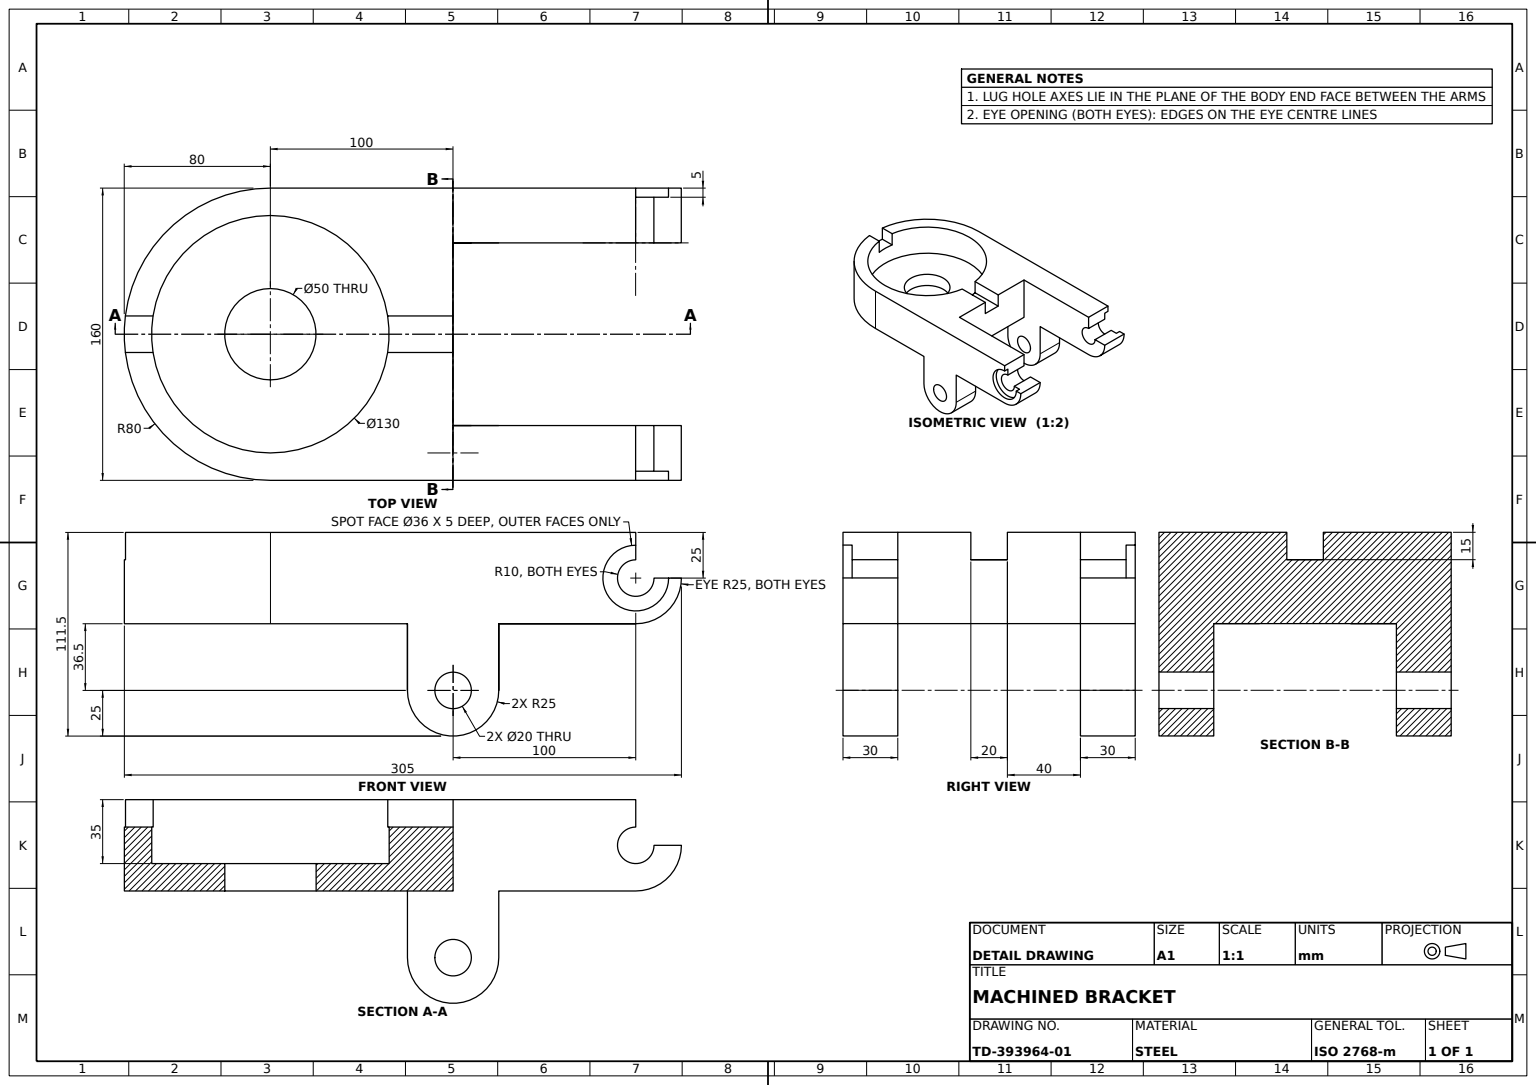
ISO-10303-21;
HEADER;
FILE_DESCRIPTION((''),'2;1');
FILE_NAME('','',(''),(''),'','','');
FILE_SCHEMA(('AUTOMOTIVE_DESIGN'));
ENDSEC;
DATA;
#1=APPLICATION_CONTEXT('');
#2=PRODUCT_CONTEXT('',#1,'mechanical');
#3=PRODUCT('','','',(#2));
#4=PRODUCT_DEFINITION_FORMATION('','',#3);
#5=PRODUCT_DEFINITION_CONTEXT('',#1,'design');
#6=PRODUCT_DEFINITION('','',#4,#5);
#7=PRODUCT_DEFINITION_SHAPE('','',#6);
#8=(LENGTH_UNIT()NAMED_UNIT(*)SI_UNIT(.MILLI.,.METRE.));
#9=(NAMED_UNIT(*)PLANE_ANGLE_UNIT()SI_UNIT($,.RADIAN.));
#10=(NAMED_UNIT(*)SI_UNIT($,.STERADIAN.)SOLID_ANGLE_UNIT());
#11=UNCERTAINTY_MEASURE_WITH_UNIT(LENGTH_MEASURE(1.E-05),#8,'distance_accuracy_value','');
#12=(GEOMETRIC_REPRESENTATION_CONTEXT(3)GLOBAL_UNCERTAINTY_ASSIGNED_CONTEXT((#11))GLOBAL_UNIT_ASSIGNED_CONTEXT((#8,#9,#10))REPRESENTATION_CONTEXT('',''));
#13=CARTESIAN_POINT('',(75.,-35.,50.));
#14=VERTEX_POINT('',#13);
#15=CARTESIAN_POINT('',(100.,-35.,50.));
#16=VERTEX_POINT('',#15);
#17=CARTESIAN_POINT('',(0.,-35.,50.));
#18=DIRECTION('',(1.,0.,0.));
#19=VECTOR('',#18,1000.);
#20=LINE('',#17,#19);
#21=EDGE_CURVE('',#14,#16,#20,.T.);
#22=ORIENTED_EDGE('',*,*,#21,.F.);
#23=CARTESIAN_POINT('',(75.,-35.,80.));
#24=VERTEX_POINT('',#23);
#25=DIRECTION('',(0.,0.,1.));
#26=VECTOR('',#25,1000.);
#27=LINE('',#13,#26);
#28=EDGE_CURVE('',#14,#24,#27,.T.);
#29=ORIENTED_EDGE('',*,*,#28,.T.);
#30=CARTESIAN_POINT('',(0.,-35.,80.));
#31=VERTEX_POINT('',#30);
#32=DIRECTION('',(-1.,0.,0.));
#33=VECTOR('',#32,1000.);
#34=LINE('',#30,#33);
#35=EDGE_CURVE('',#24,#31,#34,.T.);
#36=ORIENTED_EDGE('',*,*,#35,.T.);
#37=CARTESIAN_POINT('',(0.,-35.,-80.));
#38=VERTEX_POINT('',#37);
#39=CARTESIAN_POINT('',(0.,-35.,0.));
#40=DIRECTION('',(0.,-1.,0.));
#41=DIRECTION('',(0.,0.,-1.));
#42=AXIS2_PLACEMENT_3D('',#39,#40,#41);
#43=CIRCLE('',#42,80.);
#44=EDGE_CURVE('',#31,#38,#43,.T.);
#45=ORIENTED_EDGE('',*,*,#44,.T.);
#46=CARTESIAN_POINT('',(75.,-35.,-80.));
#47=VERTEX_POINT('',#46);
#48=LINE('',#37,#33);
#49=EDGE_CURVE('',#47,#38,#48,.T.);
#50=ORIENTED_EDGE('',*,*,#49,.F.);
#51=CARTESIAN_POINT('',(75.,-35.,-50.));
#52=VERTEX_POINT('',#51);
#53=VECTOR('',#41,1000.);
#54=LINE('',#51,#53);
#55=EDGE_CURVE('',#52,#47,#54,.T.);
#56=ORIENTED_EDGE('',*,*,#55,.F.);
#57=CARTESIAN_POINT('',(100.,-35.,-50.));
#58=VERTEX_POINT('',#57);
#59=CARTESIAN_POINT('',(0.,-35.,-50.));
#60=LINE('',#59,#19);
#61=EDGE_CURVE('',#52,#58,#60,.T.);
#62=ORIENTED_EDGE('',*,*,#61,.T.);
#63=CARTESIAN_POINT('',(100.,-35.,0.));
#64=LINE('',#63,#26);
#65=EDGE_CURVE('',#58,#16,#64,.T.);
#66=ORIENTED_EDGE('',*,*,#65,.T.);
#67=EDGE_LOOP('',(#22,#29,#36,#45,#50,#56,#62,#66));
#68=FACE_OUTER_BOUND('',#67,.T.);
#69=CARTESIAN_POINT('',(0.,-35.,25.));
#70=VERTEX_POINT('',#69);
#71=CARTESIAN_POINT('',(0.,-35.,-25.));
#72=VERTEX_POINT('',#71);
#73=CIRCLE('',#42,25.);
#74=EDGE_CURVE('',#70,#72,#73,.T.);
#75=ORIENTED_EDGE('',*,*,#74,.F.);
#76=EDGE_CURVE('',#72,#70,#73,.T.);
#77=ORIENTED_EDGE('',*,*,#76,.F.);
#78=EDGE_LOOP('',(#75,#77));
#79=FACE_BOUND('',#78,.T.);
#80=PLANE('',#42);
#81=ADVANCED_FACE('',(#68,#79),#80,.T.);
#82=CARTESIAN_POINT('',(0.,-20.,-65.));
#83=VERTEX_POINT('',#82);
#84=CARTESIAN_POINT('',(0.,-20.,65.));
#85=VERTEX_POINT('',#84);
#86=CARTESIAN_POINT('',(0.,-20.,0.));
#87=AXIS2_PLACEMENT_3D('',#86,#40,#41);
#88=CIRCLE('',#87,65.);
#89=EDGE_CURVE('',#83,#85,#88,.T.);
#90=ORIENTED_EDGE('',*,*,#89,.T.);
#91=CARTESIAN_POINT('',(0.,15.,65.));
#92=VERTEX_POINT('',#91);
#93=VECTOR('',#40,1000.);
#94=LINE('',#91,#93);
#95=EDGE_CURVE('',#92,#85,#94,.T.);
#96=ORIENTED_EDGE('',*,*,#95,.F.);
#97=CARTESIAN_POINT('',(64.226163,15.,10.));
#98=VERTEX_POINT('',#97);
#99=CARTESIAN_POINT('',(0.,15.,0.));
#100=DIRECTION('',(0.,1.,0.));
#101=AXIS2_PLACEMENT_3D('',#99,#100,#25);
#102=CIRCLE('',#101,65.);
#103=EDGE_CURVE('',#92,#98,#102,.T.);
#104=ORIENTED_EDGE('',*,*,#103,.T.);
#105=CARTESIAN_POINT('',(64.226163,0.,10.));
#106=VERTEX_POINT('',#105);
#107=LINE('',#97,#93);
#108=EDGE_CURVE('',#98,#106,#107,.T.);
#109=ORIENTED_EDGE('',*,*,#108,.T.);
#110=CARTESIAN_POINT('',(64.226163,0.,-10.));
#111=VERTEX_POINT('',#110);
#112=CARTESIAN_POINT('',(0.,0.,0.));
#113=AXIS2_PLACEMENT_3D('',#112,#100,#41);
#114=CIRCLE('',#113,65.);
#115=EDGE_CURVE('',#106,#111,#114,.T.);
#116=ORIENTED_EDGE('',*,*,#115,.T.);
#117=CARTESIAN_POINT('',(64.226163,15.,-10.));
#118=VERTEX_POINT('',#117);
#119=LINE('',#117,#93);
#120=EDGE_CURVE('',#118,#111,#119,.T.);
#121=ORIENTED_EDGE('',*,*,#120,.F.);
#122=CARTESIAN_POINT('',(0.,15.,-65.));
#123=VERTEX_POINT('',#122);
#124=EDGE_CURVE('',#118,#123,#102,.T.);
#125=ORIENTED_EDGE('',*,*,#124,.T.);
#126=LINE('',#122,#93);
#127=EDGE_CURVE('',#123,#83,#126,.T.);
#128=ORIENTED_EDGE('',*,*,#127,.T.);
#129=EDGE_LOOP('',(#90,#96,#104,#109,#116,#121,#125,#128));
#130=FACE_OUTER_BOUND('',#129,.T.);
#131=AXIS2_PLACEMENT_3D('',#99,#40,#41);
#132=CYLINDRICAL_SURFACE('',#131,65.);
#133=ADVANCED_FACE('',(#130),#132,.F.);
#134=CARTESIAN_POINT('',(90.,-71.5,80.));
#135=VERTEX_POINT('',#134);
#136=CARTESIAN_POINT('',(110.,-71.5,80.));
#137=VERTEX_POINT('',#136);
#138=CARTESIAN_POINT('',(100.,-71.5,80.));
#139=AXIS2_PLACEMENT_3D('',#138,#25,#18);
#140=CIRCLE('',#139,10.);
#141=EDGE_CURVE('',#135,#137,#140,.T.);
#142=ORIENTED_EDGE('',*,*,#141,.F.);
#143=EDGE_CURVE('',#137,#135,#140,.T.);
#144=ORIENTED_EDGE('',*,*,#143,.F.);
#145=EDGE_LOOP('',(#142,#144));
#146=FACE_BOUND('',#145,.T.);
#147=CARTESIAN_POINT('',(0.,15.,80.));
#148=VERTEX_POINT('',#147);
#149=CARTESIAN_POINT('',(200.,15.,80.));
#150=VERTEX_POINT('',#149);
#151=LINE('',#147,#19);
#152=EDGE_CURVE('',#148,#150,#151,.T.);
#153=ORIENTED_EDGE('',*,*,#152,.F.);
#154=VECTOR('',#100,1000.);
#155=LINE('',#30,#154);
#156=EDGE_CURVE('',#31,#148,#155,.T.);
#157=ORIENTED_EDGE('',*,*,#156,.F.);
#158=ORIENTED_EDGE('',*,*,#35,.F.);
#159=CARTESIAN_POINT('',(75.,-71.5,80.));
#160=VERTEX_POINT('',#159);
#161=CARTESIAN_POINT('',(75.,0.,80.));
#162=LINE('',#161,#154);
#163=EDGE_CURVE('',#160,#24,#162,.T.);
#164=ORIENTED_EDGE('',*,*,#163,.F.);
#165=CARTESIAN_POINT('',(125.,-71.5,80.));
#166=VERTEX_POINT('',#165);
#167=CIRCLE('',#139,25.);
#168=EDGE_CURVE('',#160,#166,#167,.T.);
#169=ORIENTED_EDGE('',*,*,#168,.T.);
#170=CARTESIAN_POINT('',(125.,-35.,80.));
#171=VERTEX_POINT('',#170);
#172=CARTESIAN_POINT('',(125.,0.,80.));
#173=LINE('',#172,#93);
#174=EDGE_CURVE('',#171,#166,#173,.T.);
#175=ORIENTED_EDGE('',*,*,#174,.F.);
#176=CARTESIAN_POINT('',(200.,-35.,80.));
#177=VERTEX_POINT('',#176);
#178=EDGE_CURVE('',#177,#171,#34,.T.);
#179=ORIENTED_EDGE('',*,*,#178,.F.);
#180=CARTESIAN_POINT('',(225.,-10.,80.));
#181=VERTEX_POINT('',#180);
#182=CARTESIAN_POINT('',(200.,-10.,80.));
#183=AXIS2_PLACEMENT_3D('',#182,#25,#18);
#184=CIRCLE('',#183,25.);
#185=EDGE_CURVE('',#177,#181,#184,.T.);
#186=ORIENTED_EDGE('',*,*,#185,.T.);
#187=CARTESIAN_POINT('',(218.,-10.,80.));
#188=VERTEX_POINT('',#187);
#189=LINE('',#182,#19);
#190=EDGE_CURVE('',#188,#181,#189,.T.);
#191=ORIENTED_EDGE('',*,*,#190,.F.);
#192=CARTESIAN_POINT('',(200.,8.,80.));
#193=VERTEX_POINT('',#192);
#194=CIRCLE('',#183,18.);
#195=EDGE_CURVE('',#193,#188,#194,.T.);
#196=ORIENTED_EDGE('',*,*,#195,.F.);
#197=LINE('',#149,#93);
#198=EDGE_CURVE('',#150,#193,#197,.T.);
#199=ORIENTED_EDGE('',*,*,#198,.F.);
#200=EDGE_LOOP('',(#153,#157,#158,#164,#169,#175,#179,#186,#191,#196,#199));
#201=FACE_OUTER_BOUND('',#200,.T.);
#202=AXIS2_PLACEMENT_3D('',#30,#41,#32);
#203=PLANE('',#202);
#204=ADVANCED_FACE('',(#146,#201),#203,.F.);
#205=ORIENTED_EDGE('',*,*,#127,.F.);
#206=CARTESIAN_POINT('',(-64.226163,15.,-10.));
#207=VERTEX_POINT('',#206);
#208=EDGE_CURVE('',#123,#207,#102,.T.);
#209=ORIENTED_EDGE('',*,*,#208,.T.);
#210=CARTESIAN_POINT('',(-64.226163,0.,-10.));
#211=VERTEX_POINT('',#210);
#212=LINE('',#206,#93);
#213=EDGE_CURVE('',#207,#211,#212,.T.);
#214=ORIENTED_EDGE('',*,*,#213,.T.);
#215=CARTESIAN_POINT('',(-64.226163,0.,10.));
#216=VERTEX_POINT('',#215);
#217=EDGE_CURVE('',#211,#216,#114,.T.);
#218=ORIENTED_EDGE('',*,*,#217,.T.);
#219=CARTESIAN_POINT('',(-64.226163,15.,10.));
#220=VERTEX_POINT('',#219);
#221=LINE('',#219,#93);
#222=EDGE_CURVE('',#220,#216,#221,.T.);
#223=ORIENTED_EDGE('',*,*,#222,.F.);
#224=EDGE_CURVE('',#220,#92,#102,.T.);
#225=ORIENTED_EDGE('',*,*,#224,.T.);
#226=ORIENTED_EDGE('',*,*,#95,.T.);
#227=EDGE_CURVE('',#85,#83,#88,.T.);
#228=ORIENTED_EDGE('',*,*,#227,.T.);
#229=EDGE_LOOP('',(#205,#209,#214,#218,#223,#225,#226,#228));
#230=FACE_OUTER_BOUND('',#229,.T.);
#231=ADVANCED_FACE('',(#230),#132,.F.);
#232=CARTESIAN_POINT('',(0.,-20.,25.));
#233=VERTEX_POINT('',#232);
#234=LINE('',#232,#93);
#235=EDGE_CURVE('',#233,#70,#234,.T.);
#236=ORIENTED_EDGE('',*,*,#235,.F.);
#237=CARTESIAN_POINT('',(0.,-20.,-25.));
#238=VERTEX_POINT('',#237);
#239=CIRCLE('',#87,25.);
#240=EDGE_CURVE('',#238,#233,#239,.T.);
#241=ORIENTED_EDGE('',*,*,#240,.F.);
#242=LINE('',#237,#93);
#243=EDGE_CURVE('',#238,#72,#242,.T.);
#244=ORIENTED_EDGE('',*,*,#243,.T.);
#245=ORIENTED_EDGE('',*,*,#76,.T.);
#246=EDGE_LOOP('',(#236,#241,#244,#245));
#247=FACE_OUTER_BOUND('',#246,.T.);
#248=CYLINDRICAL_SURFACE('',#87,25.);
#249=ADVANCED_FACE('',(#247),#248,.F.);
#250=CARTESIAN_POINT('',(125.,-71.5,-80.));
#251=VERTEX_POINT('',#250);
#252=CARTESIAN_POINT('',(75.,-71.5,-80.));
#253=VERTEX_POINT('',#252);
#254=CARTESIAN_POINT('',(100.,-71.5,-80.));
#255=AXIS2_PLACEMENT_3D('',#254,#41,#32);
#256=CIRCLE('',#255,25.);
#257=EDGE_CURVE('',#251,#253,#256,.T.);
#258=ORIENTED_EDGE('',*,*,#257,.F.);
#259=CARTESIAN_POINT('',(125.,-71.5,-50.));
#260=VERTEX_POINT('',#259);
#261=LINE('',#259,#53);
#262=EDGE_CURVE('',#260,#251,#261,.T.);
#263=ORIENTED_EDGE('',*,*,#262,.F.);
#264=CARTESIAN_POINT('',(75.,-71.5,-50.));
#265=VERTEX_POINT('',#264);
#266=CARTESIAN_POINT('',(100.,-71.5,-50.));
#267=AXIS2_PLACEMENT_3D('',#266,#41,#32);
#268=CIRCLE('',#267,25.);
#269=EDGE_CURVE('',#260,#265,#268,.T.);
#270=ORIENTED_EDGE('',*,*,#269,.T.);
#271=LINE('',#264,#53);
#272=EDGE_CURVE('',#265,#253,#271,.T.);
#273=ORIENTED_EDGE('',*,*,#272,.T.);
#274=EDGE_LOOP('',(#258,#263,#270,#273));
#275=FACE_OUTER_BOUND('',#274,.T.);
#276=CYLINDRICAL_SURFACE('',#267,25.);
#277=ADVANCED_FACE('',(#275),#276,.T.);
#278=CARTESIAN_POINT('',(90.,-71.5,50.));
#279=VERTEX_POINT('',#278);
#280=LINE('',#278,#26);
#281=EDGE_CURVE('',#279,#135,#280,.T.);
#282=ORIENTED_EDGE('',*,*,#281,.F.);
#283=CARTESIAN_POINT('',(110.,-71.5,50.));
#284=VERTEX_POINT('',#283);
#285=CARTESIAN_POINT('',(100.,-71.5,50.));
#286=AXIS2_PLACEMENT_3D('',#285,#25,#18);
#287=CIRCLE('',#286,10.);
#288=EDGE_CURVE('',#284,#279,#287,.T.);
#289=ORIENTED_EDGE('',*,*,#288,.F.);
#290=LINE('',#283,#26);
#291=EDGE_CURVE('',#284,#137,#290,.T.);
#292=ORIENTED_EDGE('',*,*,#291,.T.);
#293=ORIENTED_EDGE('',*,*,#143,.T.);
#294=EDGE_LOOP('',(#282,#289,#292,#293));
#295=FACE_OUTER_BOUND('',#294,.T.);
#296=CYLINDRICAL_SURFACE('',#286,10.);
#297=ADVANCED_FACE('',(#295),#296,.F.);
#298=CARTESIAN_POINT('',(125.,-35.,-50.));
#299=VERTEX_POINT('',#298);
#300=CARTESIAN_POINT('',(125.,-35.,-80.));
#301=VERTEX_POINT('',#300);
#302=LINE('',#298,#53);
#303=EDGE_CURVE('',#299,#301,#302,.T.);
#304=ORIENTED_EDGE('',*,*,#303,.T.);
#305=CARTESIAN_POINT('',(200.,-35.,-80.));
#306=VERTEX_POINT('',#305);
#307=EDGE_CURVE('',#306,#301,#48,.T.);
#308=ORIENTED_EDGE('',*,*,#307,.F.);
#309=CARTESIAN_POINT('',(200.,-35.,-50.));
#310=VERTEX_POINT('',#309);
#311=CARTESIAN_POINT('',(200.,-35.,0.));
#312=LINE('',#311,#53);
#313=EDGE_CURVE('',#310,#306,#312,.T.);
#314=ORIENTED_EDGE('',*,*,#313,.F.);
#315=EDGE_CURVE('',#299,#310,#60,.T.);
#316=ORIENTED_EDGE('',*,*,#315,.F.);
#317=EDGE_LOOP('',(#304,#308,#314,#316));
#318=FACE_OUTER_BOUND('',#317,.T.);
#319=ADVANCED_FACE('',(#318),#80,.T.);
#320=CARTESIAN_POINT('',(100.,15.,-10.));
#321=VERTEX_POINT('',#320);
#322=CARTESIAN_POINT('',(100.,0.,-10.));
#323=VERTEX_POINT('',#322);
#324=LINE('',#320,#93);
#325=EDGE_CURVE('',#321,#323,#324,.T.);
#326=ORIENTED_EDGE('',*,*,#325,.F.);
#327=CARTESIAN_POINT('',(0.,15.,-10.));
#328=LINE('',#327,#19);
#329=EDGE_CURVE('',#118,#321,#328,.T.);
#330=ORIENTED_EDGE('',*,*,#329,.F.);
#331=ORIENTED_EDGE('',*,*,#120,.T.);
#332=CARTESIAN_POINT('',(0.,0.,-10.));
#333=LINE('',#332,#19);
#334=EDGE_CURVE('',#111,#323,#333,.T.);
#335=ORIENTED_EDGE('',*,*,#334,.T.);
#336=EDGE_LOOP('',(#326,#330,#331,#335));
#337=FACE_OUTER_BOUND('',#336,.T.);
#338=AXIS2_PLACEMENT_3D('',#327,#41,#32);
#339=PLANE('',#338);
#340=ADVANCED_FACE('',(#337),#339,.F.);
#341=CARTESIAN_POINT('',(225.,-10.,-80.));
#342=VERTEX_POINT('',#341);
#343=CARTESIAN_POINT('',(200.,-10.,-80.));
#344=AXIS2_PLACEMENT_3D('',#343,#41,#32);
#345=CIRCLE('',#344,25.);
#346=EDGE_CURVE('',#342,#306,#345,.T.);
#347=ORIENTED_EDGE('',*,*,#346,.F.);
#348=CARTESIAN_POINT('',(225.,-10.,-50.));
#349=VERTEX_POINT('',#348);
#350=LINE('',#348,#53);
#351=EDGE_CURVE('',#349,#342,#350,.T.);
#352=ORIENTED_EDGE('',*,*,#351,.F.);
#353=CARTESIAN_POINT('',(200.,-10.,-50.));
#354=AXIS2_PLACEMENT_3D('',#353,#41,#32);
#355=CIRCLE('',#354,25.);
#356=EDGE_CURVE('',#349,#310,#355,.T.);
#357=ORIENTED_EDGE('',*,*,#356,.T.);
#358=ORIENTED_EDGE('',*,*,#313,.T.);
#359=EDGE_LOOP('',(#347,#352,#357,#358));
#360=FACE_OUTER_BOUND('',#359,.T.);
#361=CYLINDRICAL_SURFACE('',#354,25.);
#362=ADVANCED_FACE('',(#360),#361,.T.);
#363=CARTESIAN_POINT('',(210.,-10.,-50.));
#364=VERTEX_POINT('',#363);
#365=CARTESIAN_POINT('',(210.,-10.,-75.));
#366=VERTEX_POINT('',#365);
#367=LINE('',#363,#53);
#368=EDGE_CURVE('',#364,#366,#367,.T.);
#369=ORIENTED_EDGE('',*,*,#368,.T.);
#370=CARTESIAN_POINT('',(200.,0.,-75.));
#371=VERTEX_POINT('',#370);
#372=CARTESIAN_POINT('',(200.,-10.,-75.));
#373=AXIS2_PLACEMENT_3D('',#372,#25,#32);
#374=CIRCLE('',#373,10.);
#375=EDGE_CURVE('',#371,#366,#374,.T.);
#376=ORIENTED_EDGE('',*,*,#375,.F.);
#377=CARTESIAN_POINT('',(200.,0.,-50.));
#378=VERTEX_POINT('',#377);
#379=CARTESIAN_POINT('',(200.,0.,-120.));
#380=LINE('',#379,#26);
#381=EDGE_CURVE('',#371,#378,#380,.T.);
#382=ORIENTED_EDGE('',*,*,#381,.T.);
#383=AXIS2_PLACEMENT_3D('',#353,#25,#18);
#384=CIRCLE('',#383,10.);
#385=EDGE_CURVE('',#378,#364,#384,.T.);
#386=ORIENTED_EDGE('',*,*,#385,.T.);
#387=EDGE_LOOP('',(#369,#376,#382,#386));
#388=FACE_OUTER_BOUND('',#387,.T.);
#389=CARTESIAN_POINT('',(200.,-10.,-120.));
#390=AXIS2_PLACEMENT_3D('',#389,#25,#18);
#391=CYLINDRICAL_SURFACE('',#390,10.);
#392=ADVANCED_FACE('',(#388),#391,.F.);
#393=ORIENTED_EDGE('',*,*,#243,.F.);
#394=EDGE_CURVE('',#233,#238,#239,.T.);
#395=ORIENTED_EDGE('',*,*,#394,.F.);
#396=ORIENTED_EDGE('',*,*,#235,.T.);
#397=ORIENTED_EDGE('',*,*,#74,.T.);
#398=EDGE_LOOP('',(#393,#395,#396,#397));
#399=FACE_OUTER_BOUND('',#398,.T.);
#400=ADVANCED_FACE('',(#399),#248,.F.);
#401=ORIENTED_EDGE('',*,*,#108,.F.);
#402=CARTESIAN_POINT('',(100.,15.,10.));
#403=VERTEX_POINT('',#402);
#404=CARTESIAN_POINT('',(0.,15.,10.));
#405=LINE('',#404,#19);
#406=EDGE_CURVE('',#98,#403,#405,.T.);
#407=ORIENTED_EDGE('',*,*,#406,.T.);
#408=CARTESIAN_POINT('',(100.,0.,10.));
#409=VERTEX_POINT('',#408);
#410=LINE('',#402,#93);
#411=EDGE_CURVE('',#403,#409,#410,.T.);
#412=ORIENTED_EDGE('',*,*,#411,.T.);
#413=CARTESIAN_POINT('',(0.,0.,10.));
#414=LINE('',#413,#19);
#415=EDGE_CURVE('',#106,#409,#414,.T.);
#416=ORIENTED_EDGE('',*,*,#415,.F.);
#417=EDGE_LOOP('',(#401,#407,#412,#416));
#418=FACE_OUTER_BOUND('',#417,.T.);
#419=AXIS2_PLACEMENT_3D('',#404,#41,#32);
#420=PLANE('',#419);
#421=ADVANCED_FACE('',(#418),#420,.T.);
#422=CARTESIAN_POINT('',(200.,0.,75.));
#423=VERTEX_POINT('',#422);
#424=CARTESIAN_POINT('',(200.,8.,75.));
#425=VERTEX_POINT('',#424);
#426=CARTESIAN_POINT('',(200.,15.,75.));
#427=LINE('',#426,#154);
#428=EDGE_CURVE('',#423,#425,#427,.T.);
#429=ORIENTED_EDGE('',*,*,#428,.F.);
#430=CARTESIAN_POINT('',(200.,0.,50.));
#431=VERTEX_POINT('',#430);
#432=EDGE_CURVE('',#431,#423,#380,.T.);
#433=ORIENTED_EDGE('',*,*,#432,.F.);
#434=CARTESIAN_POINT('',(200.,15.,50.));
#435=VERTEX_POINT('',#434);
#436=CARTESIAN_POINT('',(200.,-35.,50.));
#437=LINE('',#436,#93);
#438=EDGE_CURVE('',#435,#431,#437,.T.);
#439=ORIENTED_EDGE('',*,*,#438,.F.);
#440=CARTESIAN_POINT('',(200.,15.,0.));
#441=LINE('',#440,#26);
#442=EDGE_CURVE('',#435,#150,#441,.T.);
#443=ORIENTED_EDGE('',*,*,#442,.T.);
#444=ORIENTED_EDGE('',*,*,#198,.T.);
#445=LINE('',#424,#53);
#446=EDGE_CURVE('',#193,#425,#445,.T.);
#447=ORIENTED_EDGE('',*,*,#446,.T.);
#448=EDGE_LOOP('',(#429,#433,#439,#443,#444,#447));
#449=FACE_OUTER_BOUND('',#448,.T.);
#450=CARTESIAN_POINT('',(200.,15.,-120.));
#451=AXIS2_PLACEMENT_3D('',#450,#32,#25);
#452=PLANE('',#451);
#453=ADVANCED_FACE('',(#449),#452,.F.);
#454=CARTESIAN_POINT('',(218.,-10.,-75.));
#455=VERTEX_POINT('',#454);
#456=LINE('',#365,#33);
#457=EDGE_CURVE('',#455,#366,#456,.T.);
#458=ORIENTED_EDGE('',*,*,#457,.T.);
#459=ORIENTED_EDGE('',*,*,#368,.F.);
#460=LINE('',#363,#19);
#461=EDGE_CURVE('',#364,#349,#460,.T.);
#462=ORIENTED_EDGE('',*,*,#461,.T.);
#463=ORIENTED_EDGE('',*,*,#351,.T.);
#464=CARTESIAN_POINT('',(218.,-10.,-80.));
#465=VERTEX_POINT('',#464);
#466=CARTESIAN_POINT('',(210.,-10.,-80.));
#467=LINE('',#466,#19);
#468=EDGE_CURVE('',#465,#342,#467,.T.);
#469=ORIENTED_EDGE('',*,*,#468,.F.);
#470=LINE('',#454,#53);
#471=EDGE_CURVE('',#455,#465,#470,.T.);
#472=ORIENTED_EDGE('',*,*,#471,.F.);
#473=EDGE_LOOP('',(#458,#459,#462,#463,#469,#472));
#474=FACE_OUTER_BOUND('',#473,.T.);
#475=AXIS2_PLACEMENT_3D('',#363,#100,#32);
#476=PLANE('',#475);
#477=ADVANCED_FACE('',(#474),#476,.T.);
#478=ORIENTED_EDGE('',*,*,#222,.T.);
#479=CARTESIAN_POINT('',(-79.372539,0.,10.));
#480=VERTEX_POINT('',#479);
#481=LINE('',#413,#33);
#482=EDGE_CURVE('',#216,#480,#481,.T.);
#483=ORIENTED_EDGE('',*,*,#482,.T.);
#484=CARTESIAN_POINT('',(-79.372539,15.,10.));
#485=VERTEX_POINT('',#484);
#486=LINE('',#484,#93);
#487=EDGE_CURVE('',#485,#480,#486,.T.);
#488=ORIENTED_EDGE('',*,*,#487,.F.);
#489=LINE('',#404,#33);
#490=EDGE_CURVE('',#220,#485,#489,.T.);
#491=ORIENTED_EDGE('',*,*,#490,.F.);
#492=EDGE_LOOP('',(#478,#483,#488,#491));
#493=FACE_OUTER_BOUND('',#492,.T.);
#494=AXIS2_PLACEMENT_3D('',#404,#25,#18);
#495=PLANE('',#494);
#496=ADVANCED_FACE('',(#493),#495,.F.);
#497=ORIENTED_EDGE('',*,*,#115,.F.);
#498=ORIENTED_EDGE('',*,*,#415,.T.);
#499=CARTESIAN_POINT('',(100.,0.,0.));
#500=LINE('',#499,#26);
#501=EDGE_CURVE('',#323,#409,#500,.T.);
#502=ORIENTED_EDGE('',*,*,#501,.F.);
#503=ORIENTED_EDGE('',*,*,#334,.F.);
#504=EDGE_LOOP('',(#497,#498,#502,#503));
#505=FACE_OUTER_BOUND('',#504,.T.);
#506=AXIS2_PLACEMENT_3D('',#112,#40,#41);
#507=PLANE('',#506);
#508=ADVANCED_FACE('',(#505),#507,.F.);
#509=CARTESIAN_POINT('',(-79.372539,15.,-10.));
#510=VERTEX_POINT('',#509);
#511=EDGE_CURVE('',#510,#207,#328,.T.);
#512=ORIENTED_EDGE('',*,*,#511,.F.);
#513=CARTESIAN_POINT('',(-79.372539,0.,-10.));
#514=VERTEX_POINT('',#513);
#515=LINE('',#509,#93);
#516=EDGE_CURVE('',#510,#514,#515,.T.);
#517=ORIENTED_EDGE('',*,*,#516,.T.);
#518=EDGE_CURVE('',#514,#211,#333,.T.);
#519=ORIENTED_EDGE('',*,*,#518,.T.);
#520=ORIENTED_EDGE('',*,*,#213,.F.);
#521=EDGE_LOOP('',(#512,#517,#519,#520));
#522=FACE_OUTER_BOUND('',#521,.T.);
#523=ADVANCED_FACE('',(#522),#339,.F.);
#524=ORIENTED_EDGE('',*,*,#240,.T.);
#525=ORIENTED_EDGE('',*,*,#394,.T.);
#526=EDGE_LOOP('',(#524,#525));
#527=FACE_BOUND('',#526,.T.);
#528=ORIENTED_EDGE('',*,*,#89,.F.);
#529=ORIENTED_EDGE('',*,*,#227,.F.);
#530=EDGE_LOOP('',(#528,#529));
#531=FACE_OUTER_BOUND('',#530,.T.);
#532=PLANE('',#87);
#533=ADVANCED_FACE('',(#527,#531),#532,.F.);
#534=ORIENTED_EDGE('',*,*,#516,.F.);
#535=CARTESIAN_POINT('',(0.,15.,-80.));
#536=VERTEX_POINT('',#535);
#537=CIRCLE('',#101,80.);
#538=EDGE_CURVE('',#536,#510,#537,.T.);
#539=ORIENTED_EDGE('',*,*,#538,.F.);
#540=LINE('',#535,#93);
#541=EDGE_CURVE('',#536,#38,#540,.T.);
#542=ORIENTED_EDGE('',*,*,#541,.T.);
#543=ORIENTED_EDGE('',*,*,#44,.F.);
#544=ORIENTED_EDGE('',*,*,#156,.T.);
#545=EDGE_CURVE('',#485,#148,#537,.T.);
#546=ORIENTED_EDGE('',*,*,#545,.F.);
#547=ORIENTED_EDGE('',*,*,#487,.T.);
#548=CIRCLE('',#506,80.);
#549=EDGE_CURVE('',#480,#514,#548,.T.);
#550=ORIENTED_EDGE('',*,*,#549,.T.);
#551=EDGE_LOOP('',(#534,#539,#542,#543,#544,#546,#547,#550));
#552=FACE_OUTER_BOUND('',#551,.T.);
#553=CYLINDRICAL_SURFACE('',#131,80.);
#554=ADVANCED_FACE('',(#552),#553,.T.);
#555=CARTESIAN_POINT('',(125.,-71.5,50.));
#556=VERTEX_POINT('',#555);
#557=LINE('',#555,#26);
#558=EDGE_CURVE('',#556,#166,#557,.T.);
#559=ORIENTED_EDGE('',*,*,#558,.F.);
#560=CARTESIAN_POINT('',(125.,-35.,50.));
#561=VERTEX_POINT('',#560);
#562=CARTESIAN_POINT('',(125.,0.,50.));
#563=LINE('',#562,#93);
#564=EDGE_CURVE('',#561,#556,#563,.T.);
#565=ORIENTED_EDGE('',*,*,#564,.F.);
#566=LINE('',#560,#26);
#567=EDGE_CURVE('',#561,#171,#566,.T.);
#568=ORIENTED_EDGE('',*,*,#567,.T.);
#569=ORIENTED_EDGE('',*,*,#174,.T.);
#570=EDGE_LOOP('',(#559,#565,#568,#569));
#571=FACE_OUTER_BOUND('',#570,.T.);
#572=AXIS2_PLACEMENT_3D('',#562,#32,#25);
#573=PLANE('',#572);
#574=ADVANCED_FACE('',(#571),#573,.F.);
#575=CARTESIAN_POINT('',(200.,8.,-80.));
#576=VERTEX_POINT('',#575);
#577=CARTESIAN_POINT('',(200.,8.,-75.));
#578=VERTEX_POINT('',#577);
#579=LINE('',#577,#26);
#580=EDGE_CURVE('',#576,#578,#579,.T.);
#581=ORIENTED_EDGE('',*,*,#580,.T.);
#582=CARTESIAN_POINT('',(182.,-10.,-75.));
#583=VERTEX_POINT('',#582);
#584=AXIS2_PLACEMENT_3D('',#372,#41,#32);
#585=CIRCLE('',#584,18.);
#586=EDGE_CURVE('',#583,#578,#585,.T.);
#587=ORIENTED_EDGE('',*,*,#586,.F.);
#588=CARTESIAN_POINT('',(182.,-10.,-80.));
#589=VERTEX_POINT('',#588);
#590=LINE('',#582,#53);
#591=EDGE_CURVE('',#583,#589,#590,.T.);
#592=ORIENTED_EDGE('',*,*,#591,.T.);
#593=CIRCLE('',#344,18.);
#594=EDGE_CURVE('',#589,#576,#593,.T.);
#595=ORIENTED_EDGE('',*,*,#594,.T.);
#596=EDGE_LOOP('',(#581,#587,#592,#595));
#597=FACE_OUTER_BOUND('',#596,.T.);
#598=CYLINDRICAL_SURFACE('',#584,18.);
#599=ADVANCED_FACE('',(#597),#598,.F.);
#600=ORIENTED_EDGE('',*,*,#217,.F.);
#601=ORIENTED_EDGE('',*,*,#518,.F.);
#602=ORIENTED_EDGE('',*,*,#549,.F.);
#603=ORIENTED_EDGE('',*,*,#482,.F.);
#604=EDGE_LOOP('',(#600,#601,#602,#603));
#605=FACE_OUTER_BOUND('',#604,.T.);
#606=ADVANCED_FACE('',(#605),#507,.F.);
#607=CARTESIAN_POINT('',(218.,-10.,75.));
#608=VERTEX_POINT('',#607);
#609=CARTESIAN_POINT('',(200.,-10.,75.));
#610=AXIS2_PLACEMENT_3D('',#609,#25,#18);
#611=CIRCLE('',#610,18.);
#612=EDGE_CURVE('',#425,#608,#611,.T.);
#613=ORIENTED_EDGE('',*,*,#612,.T.);
#614=CARTESIAN_POINT('',(210.,-10.,75.));
#615=VERTEX_POINT('',#614);
#616=LINE('',#609,#33);
#617=EDGE_CURVE('',#608,#615,#616,.T.);
#618=ORIENTED_EDGE('',*,*,#617,.T.);
#619=AXIS2_PLACEMENT_3D('',#609,#41,#18);
#620=CIRCLE('',#619,10.);
#621=EDGE_CURVE('',#615,#423,#620,.T.);
#622=ORIENTED_EDGE('',*,*,#621,.T.);
#623=ORIENTED_EDGE('',*,*,#428,.T.);
#624=EDGE_LOOP('',(#613,#618,#622,#623));
#625=FACE_OUTER_BOUND('',#624,.T.);
#626=PLANE('',#610);
#627=ADVANCED_FACE('',(#625),#626,.T.);
#628=CARTESIAN_POINT('',(75.,0.,-50.));
#629=LINE('',#628,#93);
#630=EDGE_CURVE('',#52,#265,#629,.T.);
#631=ORIENTED_EDGE('',*,*,#630,.F.);
#632=ORIENTED_EDGE('',*,*,#55,.T.);
#633=CARTESIAN_POINT('',(75.,0.,-80.));
#634=LINE('',#633,#93);
#635=EDGE_CURVE('',#47,#253,#634,.T.);
#636=ORIENTED_EDGE('',*,*,#635,.T.);
#637=ORIENTED_EDGE('',*,*,#272,.F.);
#638=EDGE_LOOP('',(#631,#632,#636,#637));
#639=FACE_OUTER_BOUND('',#638,.T.);
#640=AXIS2_PLACEMENT_3D('',#628,#18,#41);
#641=PLANE('',#640);
#642=ADVANCED_FACE('',(#639),#641,.F.);
#643=CARTESIAN_POINT('',(100.,15.,50.));
#644=VERTEX_POINT('',#643);
#645=CARTESIAN_POINT('',(100.,15.,0.));
#646=LINE('',#645,#26);
#647=EDGE_CURVE('',#403,#644,#646,.T.);
#648=ORIENTED_EDGE('',*,*,#647,.F.);
#649=ORIENTED_EDGE('',*,*,#406,.F.);
#650=ORIENTED_EDGE('',*,*,#103,.F.);
#651=ORIENTED_EDGE('',*,*,#224,.F.);
#652=ORIENTED_EDGE('',*,*,#490,.T.);
#653=ORIENTED_EDGE('',*,*,#545,.T.);
#654=ORIENTED_EDGE('',*,*,#152,.T.);
#655=ORIENTED_EDGE('',*,*,#442,.F.);
#656=CARTESIAN_POINT('',(0.,15.,50.));
#657=LINE('',#656,#19);
#658=EDGE_CURVE('',#644,#435,#657,.T.);
#659=ORIENTED_EDGE('',*,*,#658,.F.);
#660=EDGE_LOOP('',(#648,#649,#650,#651,#652,#653,#654,#655,#659));
#661=FACE_OUTER_BOUND('',#660,.T.);
#662=PLANE('',#101);
#663=ADVANCED_FACE('',(#661),#662,.T.);
#664=CARTESIAN_POINT('',(75.,-71.5,50.));
#665=VERTEX_POINT('',#664);
#666=LINE('',#664,#26);
#667=EDGE_CURVE('',#665,#160,#666,.T.);
#668=ORIENTED_EDGE('',*,*,#667,.T.);
#669=ORIENTED_EDGE('',*,*,#163,.T.);
#670=ORIENTED_EDGE('',*,*,#28,.F.);
#671=CARTESIAN_POINT('',(75.,0.,50.));
#672=LINE('',#671,#154);
#673=EDGE_CURVE('',#665,#14,#672,.T.);
#674=ORIENTED_EDGE('',*,*,#673,.F.);
#675=EDGE_LOOP('',(#668,#669,#670,#674));
#676=FACE_OUTER_BOUND('',#675,.T.);
#677=AXIS2_PLACEMENT_3D('',#671,#18,#41);
#678=PLANE('',#677);
#679=ADVANCED_FACE('',(#676),#678,.F.);
#680=EDGE_CURVE('',#455,#583,#585,.T.);
#681=ORIENTED_EDGE('',*,*,#680,.F.);
#682=ORIENTED_EDGE('',*,*,#471,.T.);
#683=EDGE_CURVE('',#465,#589,#593,.T.);
#684=ORIENTED_EDGE('',*,*,#683,.T.);
#685=ORIENTED_EDGE('',*,*,#591,.F.);
#686=EDGE_LOOP('',(#681,#682,#684,#685));
#687=FACE_OUTER_BOUND('',#686,.T.);
#688=ADVANCED_FACE('',(#687),#598,.F.);
#689=CARTESIAN_POINT('',(200.,15.,-80.));
#690=VERTEX_POINT('',#689);
#691=CARTESIAN_POINT('',(200.,15.,-50.));
#692=VERTEX_POINT('',#691);
#693=EDGE_CURVE('',#690,#692,#441,.T.);
#694=ORIENTED_EDGE('',*,*,#693,.T.);
#695=LINE('',#691,#93);
#696=EDGE_CURVE('',#692,#378,#695,.T.);
#697=ORIENTED_EDGE('',*,*,#696,.T.);
#698=ORIENTED_EDGE('',*,*,#381,.F.);
#699=CARTESIAN_POINT('',(200.,15.,-75.));
#700=LINE('',#699,#154);
#701=EDGE_CURVE('',#371,#578,#700,.T.);
#702=ORIENTED_EDGE('',*,*,#701,.T.);
#703=ORIENTED_EDGE('',*,*,#580,.F.);
#704=LINE('',#689,#93);
#705=EDGE_CURVE('',#690,#576,#704,.T.);
#706=ORIENTED_EDGE('',*,*,#705,.F.);
#707=EDGE_LOOP('',(#694,#697,#698,#702,#703,#706));
#708=FACE_OUTER_BOUND('',#707,.T.);
#709=AXIS2_PLACEMENT_3D('',#440,#18,#41);
#710=PLANE('',#709);
#711=ADVANCED_FACE('',(#708),#710,.T.);
#712=CARTESIAN_POINT('',(110.,-71.5,-50.));
#713=VERTEX_POINT('',#712);
#714=CARTESIAN_POINT('',(90.,-71.5,-50.));
#715=VERTEX_POINT('',#714);
#716=CIRCLE('',#267,10.);
#717=EDGE_CURVE('',#713,#715,#716,.T.);
#718=ORIENTED_EDGE('',*,*,#717,.T.);
#719=EDGE_CURVE('',#715,#713,#716,.T.);
#720=ORIENTED_EDGE('',*,*,#719,.T.);
#721=EDGE_LOOP('',(#718,#720));
#722=FACE_BOUND('',#721,.T.);
#723=ORIENTED_EDGE('',*,*,#315,.T.);
#724=ORIENTED_EDGE('',*,*,#356,.F.);
#725=ORIENTED_EDGE('',*,*,#461,.F.);
#726=ORIENTED_EDGE('',*,*,#385,.F.);
#727=ORIENTED_EDGE('',*,*,#696,.F.);
#728=CARTESIAN_POINT('',(100.,15.,-50.));
#729=VERTEX_POINT('',#728);
#730=CARTESIAN_POINT('',(0.,15.,-50.));
#731=LINE('',#730,#33);
#732=EDGE_CURVE('',#692,#729,#731,.T.);
#733=ORIENTED_EDGE('',*,*,#732,.T.);
#734=LINE('',#728,#93);
#735=EDGE_CURVE('',#729,#58,#734,.T.);
#736=ORIENTED_EDGE('',*,*,#735,.T.);
#737=ORIENTED_EDGE('',*,*,#61,.F.);
#738=ORIENTED_EDGE('',*,*,#630,.T.);
#739=ORIENTED_EDGE('',*,*,#269,.F.);
#740=CARTESIAN_POINT('',(125.,0.,-50.));
#741=LINE('',#740,#154);
#742=EDGE_CURVE('',#260,#299,#741,.T.);
#743=ORIENTED_EDGE('',*,*,#742,.T.);
#744=EDGE_LOOP('',(#723,#724,#725,#726,#727,#733,#736,#737,#738,#739,#743));
#745=FACE_OUTER_BOUND('',#744,.T.);
#746=AXIS2_PLACEMENT_3D('',#730,#25,#18);
#747=PLANE('',#746);
#748=ADVANCED_FACE('',(#722,#745),#747,.T.);
#749=EDGE_CURVE('',#279,#284,#287,.T.);
#750=ORIENTED_EDGE('',*,*,#749,.T.);
#751=ORIENTED_EDGE('',*,*,#288,.T.);
#752=EDGE_LOOP('',(#750,#751));
#753=FACE_BOUND('',#752,.T.);
#754=ORIENTED_EDGE('',*,*,#673,.T.);
#755=ORIENTED_EDGE('',*,*,#21,.T.);
#756=LINE('',#15,#154);
#757=EDGE_CURVE('',#16,#644,#756,.T.);
#758=ORIENTED_EDGE('',*,*,#757,.T.);
#759=ORIENTED_EDGE('',*,*,#658,.T.);
#760=ORIENTED_EDGE('',*,*,#438,.T.);
#761=CARTESIAN_POINT('',(210.,-10.,50.));
#762=VERTEX_POINT('',#761);
#763=CARTESIAN_POINT('',(200.,-10.,50.));
#764=AXIS2_PLACEMENT_3D('',#763,#25,#18);
#765=CIRCLE('',#764,10.);
#766=EDGE_CURVE('',#431,#762,#765,.T.);
#767=ORIENTED_EDGE('',*,*,#766,.T.);
#768=CARTESIAN_POINT('',(225.,-10.,50.));
#769=VERTEX_POINT('',#768);
#770=CARTESIAN_POINT('',(0.,-10.,50.));
#771=LINE('',#770,#19);
#772=EDGE_CURVE('',#762,#769,#771,.T.);
#773=ORIENTED_EDGE('',*,*,#772,.T.);
#774=VERTEX_POINT('',#436);
#775=CIRCLE('',#764,25.);
#776=EDGE_CURVE('',#774,#769,#775,.T.);
#777=ORIENTED_EDGE('',*,*,#776,.F.);
#778=EDGE_CURVE('',#561,#774,#20,.T.);
#779=ORIENTED_EDGE('',*,*,#778,.F.);
#780=ORIENTED_EDGE('',*,*,#564,.T.);
#781=CIRCLE('',#286,25.);
#782=EDGE_CURVE('',#665,#556,#781,.T.);
#783=ORIENTED_EDGE('',*,*,#782,.F.);
#784=EDGE_LOOP('',(#754,#755,#758,#759,#760,#767,#773,#777,#779,#780,#783));
#785=FACE_OUTER_BOUND('',#784,.T.);
#786=AXIS2_PLACEMENT_3D('',#17,#25,#18);
#787=PLANE('',#786);
#788=ADVANCED_FACE('',(#753,#785),#787,.F.);
#789=CARTESIAN_POINT('',(90.,-71.5,-80.));
#790=VERTEX_POINT('',#789);
#791=LINE('',#714,#53);
#792=EDGE_CURVE('',#715,#790,#791,.T.);
#793=ORIENTED_EDGE('',*,*,#792,.T.);
#794=CARTESIAN_POINT('',(110.,-71.5,-80.));
#795=VERTEX_POINT('',#794);
#796=CIRCLE('',#255,10.);
#797=EDGE_CURVE('',#790,#795,#796,.T.);
#798=ORIENTED_EDGE('',*,*,#797,.T.);
#799=LINE('',#712,#53);
#800=EDGE_CURVE('',#713,#795,#799,.T.);
#801=ORIENTED_EDGE('',*,*,#800,.F.);
#802=ORIENTED_EDGE('',*,*,#719,.F.);
#803=EDGE_LOOP('',(#793,#798,#801,#802));
#804=FACE_OUTER_BOUND('',#803,.T.);
#805=CYLINDRICAL_SURFACE('',#267,10.);
#806=ADVANCED_FACE('',(#804),#805,.F.);
#807=ORIENTED_EDGE('',*,*,#612,.F.);
#808=ORIENTED_EDGE('',*,*,#446,.F.);
#809=ORIENTED_EDGE('',*,*,#195,.T.);
#810=LINE('',#607,#26);
#811=EDGE_CURVE('',#608,#188,#810,.T.);
#812=ORIENTED_EDGE('',*,*,#811,.F.);
#813=EDGE_LOOP('',(#807,#808,#809,#812));
#814=FACE_OUTER_BOUND('',#813,.T.);
#815=CYLINDRICAL_SURFACE('',#610,18.);
#816=ADVANCED_FACE('',(#814),#815,.F.);
#817=EDGE_CURVE('',#795,#790,#796,.T.);
#818=ORIENTED_EDGE('',*,*,#817,.T.);
#819=ORIENTED_EDGE('',*,*,#792,.F.);
#820=ORIENTED_EDGE('',*,*,#717,.F.);
#821=ORIENTED_EDGE('',*,*,#800,.T.);
#822=EDGE_LOOP('',(#818,#819,#820,#821));
#823=FACE_OUTER_BOUND('',#822,.T.);
#824=ADVANCED_FACE('',(#823),#805,.F.);
#825=ORIENTED_EDGE('',*,*,#817,.F.);
#826=ORIENTED_EDGE('',*,*,#797,.F.);
#827=EDGE_LOOP('',(#825,#826));
#828=FACE_BOUND('',#827,.T.);
#829=ORIENTED_EDGE('',*,*,#594,.F.);
#830=ORIENTED_EDGE('',*,*,#683,.F.);
#831=ORIENTED_EDGE('',*,*,#468,.T.);
#832=ORIENTED_EDGE('',*,*,#346,.T.);
#833=ORIENTED_EDGE('',*,*,#307,.T.);
#834=CARTESIAN_POINT('',(125.,0.,-80.));
#835=LINE('',#834,#154);
#836=EDGE_CURVE('',#251,#301,#835,.T.);
#837=ORIENTED_EDGE('',*,*,#836,.F.);
#838=ORIENTED_EDGE('',*,*,#257,.T.);
#839=ORIENTED_EDGE('',*,*,#635,.F.);
#840=ORIENTED_EDGE('',*,*,#49,.T.);
#841=ORIENTED_EDGE('',*,*,#541,.F.);
#842=LINE('',#535,#19);
#843=EDGE_CURVE('',#536,#690,#842,.T.);
#844=ORIENTED_EDGE('',*,*,#843,.T.);
#845=ORIENTED_EDGE('',*,*,#705,.T.);
#846=EDGE_LOOP('',(#829,#830,#831,#832,#833,#837,#838,#839,#840,#841,#844,#845));
#847=FACE_OUTER_BOUND('',#846,.T.);
#848=AXIS2_PLACEMENT_3D('',#535,#41,#32);
#849=PLANE('',#848);
#850=ADVANCED_FACE('',(#828,#847),#849,.T.);
#851=ORIENTED_EDGE('',*,*,#375,.T.);
#852=ORIENTED_EDGE('',*,*,#457,.F.);
#853=ORIENTED_EDGE('',*,*,#680,.T.);
#854=ORIENTED_EDGE('',*,*,#586,.T.);
#855=ORIENTED_EDGE('',*,*,#701,.F.);
#856=EDGE_LOOP('',(#851,#852,#853,#854,#855));
#857=FACE_OUTER_BOUND('',#856,.T.);
#858=PLANE('',#584);
#859=ADVANCED_FACE('',(#857),#858,.T.);
#860=ORIENTED_EDGE('',*,*,#735,.F.);
#861=EDGE_CURVE('',#729,#321,#646,.T.);
#862=ORIENTED_EDGE('',*,*,#861,.T.);
#863=ORIENTED_EDGE('',*,*,#325,.T.);
#864=ORIENTED_EDGE('',*,*,#501,.T.);
#865=ORIENTED_EDGE('',*,*,#411,.F.);
#866=ORIENTED_EDGE('',*,*,#647,.T.);
#867=ORIENTED_EDGE('',*,*,#757,.F.);
#868=ORIENTED_EDGE('',*,*,#65,.F.);
#869=EDGE_LOOP('',(#860,#862,#863,#864,#865,#866,#867,#868));
#870=FACE_OUTER_BOUND('',#869,.T.);
#871=AXIS2_PLACEMENT_3D('',#645,#18,#41);
#872=PLANE('',#871);
#873=ADVANCED_FACE('',(#870),#872,.T.);
#874=ORIENTED_EDGE('',*,*,#617,.F.);
#875=ORIENTED_EDGE('',*,*,#811,.T.);
#876=ORIENTED_EDGE('',*,*,#190,.T.);
#877=CARTESIAN_POINT('',(225.,-10.,-120.));
#878=LINE('',#877,#26);
#879=EDGE_CURVE('',#769,#181,#878,.T.);
#880=ORIENTED_EDGE('',*,*,#879,.F.);
#881=ORIENTED_EDGE('',*,*,#772,.F.);
#882=CARTESIAN_POINT('',(210.,-10.,-120.));
#883=LINE('',#882,#53);
#884=EDGE_CURVE('',#615,#762,#883,.T.);
#885=ORIENTED_EDGE('',*,*,#884,.F.);
#886=EDGE_LOOP('',(#874,#875,#876,#880,#881,#885));
#887=FACE_OUTER_BOUND('',#886,.T.);
#888=AXIS2_PLACEMENT_3D('',#389,#40,#41);
#889=PLANE('',#888);
#890=ADVANCED_FACE('',(#887),#889,.F.);
#891=ORIENTED_EDGE('',*,*,#538,.T.);
#892=ORIENTED_EDGE('',*,*,#511,.T.);
#893=ORIENTED_EDGE('',*,*,#208,.F.);
#894=ORIENTED_EDGE('',*,*,#124,.F.);
#895=ORIENTED_EDGE('',*,*,#329,.T.);
#896=ORIENTED_EDGE('',*,*,#861,.F.);
#897=ORIENTED_EDGE('',*,*,#732,.F.);
#898=ORIENTED_EDGE('',*,*,#693,.F.);
#899=ORIENTED_EDGE('',*,*,#843,.F.);
#900=EDGE_LOOP('',(#891,#892,#893,#894,#895,#896,#897,#898,#899));
#901=FACE_OUTER_BOUND('',#900,.T.);
#902=ADVANCED_FACE('',(#901),#662,.T.);
#903=LINE('',#311,#26);
#904=EDGE_CURVE('',#774,#177,#903,.T.);
#905=ORIENTED_EDGE('',*,*,#904,.T.);
#906=ORIENTED_EDGE('',*,*,#178,.T.);
#907=ORIENTED_EDGE('',*,*,#567,.F.);
#908=ORIENTED_EDGE('',*,*,#778,.T.);
#909=EDGE_LOOP('',(#905,#906,#907,#908));
#910=FACE_OUTER_BOUND('',#909,.T.);
#911=ADVANCED_FACE('',(#910),#80,.T.);
#912=ORIENTED_EDGE('',*,*,#776,.T.);
#913=ORIENTED_EDGE('',*,*,#879,.T.);
#914=ORIENTED_EDGE('',*,*,#185,.F.);
#915=ORIENTED_EDGE('',*,*,#904,.F.);
#916=EDGE_LOOP('',(#912,#913,#914,#915));
#917=FACE_OUTER_BOUND('',#916,.T.);
#918=CYLINDRICAL_SURFACE('',#764,25.);
#919=ADVANCED_FACE('',(#917),#918,.T.);
#920=ORIENTED_EDGE('',*,*,#432,.T.);
#921=ORIENTED_EDGE('',*,*,#621,.F.);
#922=ORIENTED_EDGE('',*,*,#884,.T.);
#923=ORIENTED_EDGE('',*,*,#766,.F.);
#924=EDGE_LOOP('',(#920,#921,#922,#923));
#925=FACE_OUTER_BOUND('',#924,.T.);
#926=ADVANCED_FACE('',(#925),#391,.F.);
#927=ORIENTED_EDGE('',*,*,#782,.T.);
#928=ORIENTED_EDGE('',*,*,#558,.T.);
#929=ORIENTED_EDGE('',*,*,#168,.F.);
#930=ORIENTED_EDGE('',*,*,#667,.F.);
#931=EDGE_LOOP('',(#927,#928,#929,#930));
#932=FACE_OUTER_BOUND('',#931,.T.);
#933=CYLINDRICAL_SURFACE('',#286,25.);
#934=ADVANCED_FACE('',(#932),#933,.T.);
#935=ORIENTED_EDGE('',*,*,#303,.F.);
#936=ORIENTED_EDGE('',*,*,#742,.F.);
#937=ORIENTED_EDGE('',*,*,#262,.T.);
#938=ORIENTED_EDGE('',*,*,#836,.T.);
#939=EDGE_LOOP('',(#935,#936,#937,#938));
#940=FACE_OUTER_BOUND('',#939,.T.);
#941=AXIS2_PLACEMENT_3D('',#740,#32,#25);
#942=PLANE('',#941);
#943=ADVANCED_FACE('',(#940),#942,.F.);
#944=ORIENTED_EDGE('',*,*,#749,.F.);
#945=ORIENTED_EDGE('',*,*,#281,.T.);
#946=ORIENTED_EDGE('',*,*,#141,.T.);
#947=ORIENTED_EDGE('',*,*,#291,.F.);
#948=EDGE_LOOP('',(#944,#945,#946,#947));
#949=FACE_OUTER_BOUND('',#948,.T.);
#950=ADVANCED_FACE('',(#949),#296,.F.);
#951=CLOSED_SHELL('',(#81,#133,#204,#231,#249,#277,#297,#319,#340,#362,#392,#400,#421,#453,#477,#496,#508,#523,#533,#554,#574,#599,#606,#627,#642,#663,#679,#688,#711,#748,#788,#806,#816,#824,#850,#859,#873,#890,#902,#911,#919,#926,#934,#943,#950));
#952=MANIFOLD_SOLID_BREP('',#951);
#953=ADVANCED_BREP_SHAPE_REPRESENTATION('',(#952),#12);
#954=SHAPE_DEFINITION_REPRESENTATION(#7,#953);
ENDSEC;
END-ISO-10303-21;
